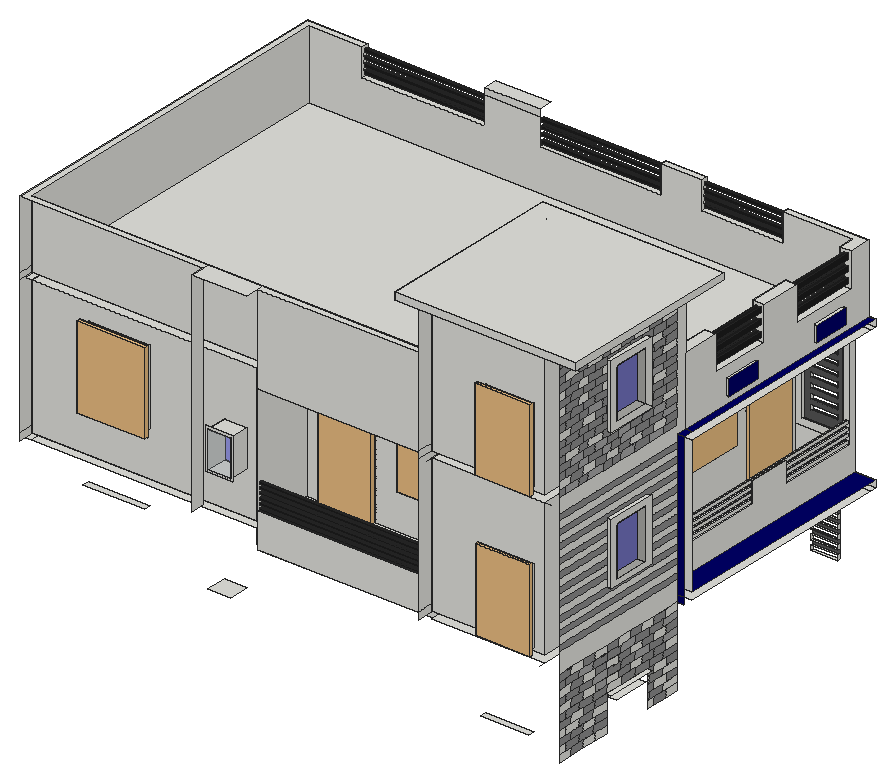
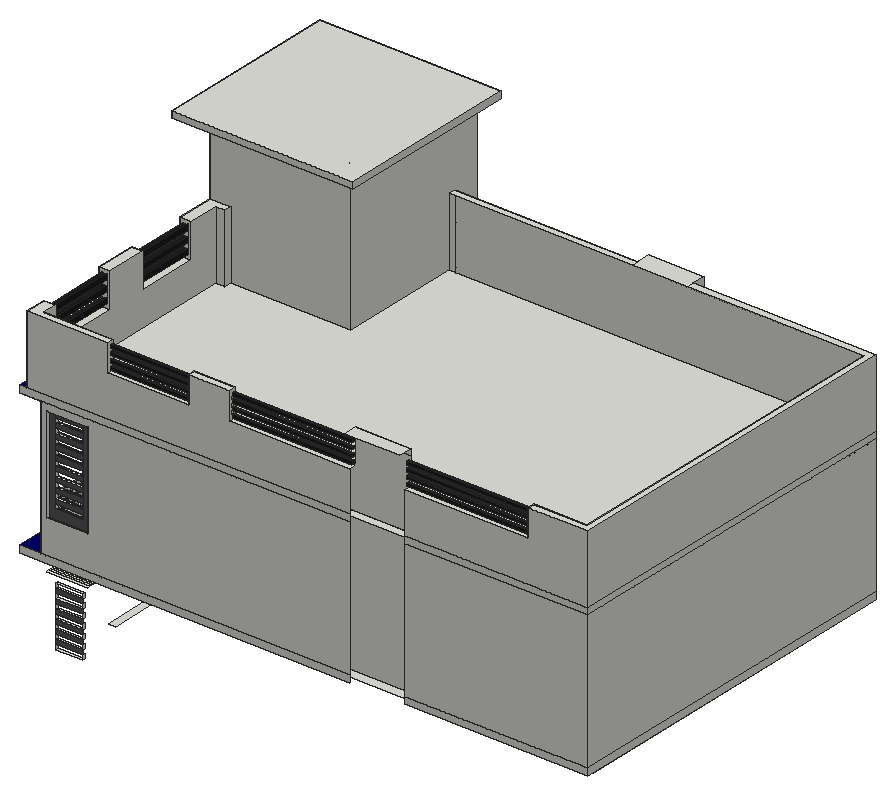
# SketchUp Ruby script. Lengths in inches.
U = 1.inch
M = Sketchup.active_model
def pt(a) = Geom::Point3d.new(a.map { |v| v * U })
def face(e, loops, mat)
  f = e.add_face(loops[0].map { |a| pt(a) })
  loops[1..].each { |l| e.add_face(l.map { |a| pt(a) }).erase! }
  f.material = f.back_material = mat if mat
  f
end
# faces: each face lists its corners as indices into pts; further lists are holes
def faces(e, pts, list, mat = nil) = list.each { |f| face(e, (f[0].is_a?(Array) ? f : [f]).map { |l| l.map { |i| pts[i] } }, mat) }
# xy, xz, yz: faces in a plane at the given z, y or x. An outline is a flat list of corners, or four numbers for a rectangle; further outlines are holes
def ring(l) = l.size == 4 ? [[l[0], l[1]], [l[2], l[1]], [l[2], l[3]], [l[0], l[3]]] : l.each_slice(2).to_a
def flat(e, list, mat, &to3) = list.each { |f| face(e, (f[0].is_a?(Array) ? f : [f]).map { |l| ring(l).map { |u, v| to3.(u, v) } }, mat) }
def xy(e, z, list, mat = nil) = flat(e, list, mat) { |x, y| [x, y, z] }
def xz(e, y, list, mat = nil) = flat(e, list, mat) { |x, z| [x, y, z] }
def yz(e, x, list, mat = nil) = flat(e, list, mat) { |y, z| [x, y, z] }
def lines(e, pts, list) = list.each { |a, b| e.add_line(pt(pts[a]), pt(pts[b])) }
# prism: a flat outline (further loops are holes) pulled along v
def prism(e, loops, v, mat = nil)
  f = face(e, loops, mat); d = Geom::Vector3d.new(v.map { |x| x * U })
  f.pushpull(f.normal.samedirection?(d) ? d.length : -d.length)
end
def box(e, o, s, mat = nil) = prism(e, [[o, [o[0] + s[0], o[1], o[2]], [o[0] + s[0], o[1] + s[1], o[2]], [o[0], o[1] + s[1], o[2]]]], [0, 0, s[2]], mat)
def at(x, y, z, deg = 0) = Geom::Transformation.translation(pt([x, y, z])) * Geom::Transformation.rotation(ORIGIN, Z_AXIS, deg.degrees)
def axes(o, x, y, z) = Geom::Transformation.new([*x, 0, *y, 0, *z, 0, *pt(o).to_a, 1])
def part(name) = M.definitions.add(name)
# library, detail: a bought-in or finely detailed component or shape, given as its bounding box
def library(name, o, s) = part(name).tap { |d| box(d.entities, o, s) }
def detail(e, o, s) = box(e.add_group.entities, o, s)
def put(e, d, t, mat = nil) = e.add_instance(d, t).tap { |i| i.material = mat if mat }
def group(e, t, mat = nil) = e.add_group.tap { |g| g.transformation = t; g.material = mat if mat }.entities
root = M.entities
M.materials.add("Glass_Basic_01").color = [0, 0, 0]
M.materials["Glass_Basic_01"].alpha = 0.25
M.materials.add("Glass_Basic_1").color = [161, 173, 186]
M.materials["Glass_Basic_1"].alpha = 0.25
M.materials.add("I02_Moonlit_Azure").color = [153, 153, 255]
M.materials.add("I08_Inkstorm").color = [0, 0, 102]
M.materials.add("M03_Pewter_Shine").color = [168, 168, 168]
M.materials.add("M04_Stone_Frost").color = [142, 142, 142]
M.materials.add("M06_Steel_Smoke").color = [86, 86, 86]
M.materials.add("M08_Obsidian_Black").color = [30, 30, 30]
c1 = library("porta+4",[0.2,-5.42,1.33],[46.55,4.72,83.21])
c2 = library("mesh-162",[-1607.75,-1245.64,-53.98],[1739.16,1702.88,120.91])
c3 = part("Group9")
put(c3.entities,c2,at(0,0,0))
c4 = part("Balcony railing")
xy(c4.entities,0.4,[[0,0.79,160.5,2.29]])
xy(c4.entities,2.4,[[0,0.79,160.5,2.29]])
xy(c4.entities,4.59,[[0,0.79,160.5,2.29]])
xy(c4.entities,6.59,[[0,0.79,160.5,2.29]])
xy(c4.entities,8.79,[[0,0.79,160.5,2.29]])
xy(c4.entities,10.79,[[0,0.79,160.5,2.29]])
xy(c4.entities,12.98,[[0,0.79,160.5,2.29]])
xy(c4.entities,14.98,[[0,0.79,160.5,2.29]])
xy(c4.entities,17.17,[[0,0.79,160.5,2.29]])
xy(c4.entities,19.17,[[0,0.79,160.5,2.29]])
xy(c4.entities,21.36,[[0,0.79,160.5,2.29]])
xy(c4.entities,23.36,[[0,0.79,160.5,2.29]])
xz(c4.entities,0.79,[[0,0.4,160.5,2.4],[0,4.59,160.5,6.59],[0,8.79,160.5,10.79],[0,12.98,160.5,14.98],[0,17.17,160.5,19.17],
  [0,21.36,160.5,23.36]])
xz(c4.entities,2.29,[[0,0.4,160.5,2.4],[0,4.59,160.5,6.59],[0,8.79,160.5,10.79],[0,12.98,160.5,14.98],[0,17.17,160.5,19.17],
  [0,21.36,160.5,23.36]])
yz(c4.entities,0,[[[0,0,3,24],[0.79,21.36,2.29,23.36],[0.79,17.17,2.29,19.17],[0.79,12.98,2.29,14.98],[0.79,8.79,2.29,10.79],[0.79,4.59,2.29,6.59],[0.79,0.4,2.29,2.4]]])
yz(c4.entities,160.5,[[0.79,0.4,2.29,2.4],[0.79,4.59,2.29,6.59],[0.79,8.79,2.29,10.79],[0.79,12.98,2.29,14.98],[0.79,17.17,2.29,19.17],
  [0.79,21.36,2.29,23.36]])
c5 = part("RAIL")
xy(c5.entities,0,[[0,0,2,195]])
xy(c5.entities,2.57,[[0,0,2,195]])
xy(c5.entities,5.14,[[0,0,2,195]])
xy(c5.entities,7.71,[[0,0,2,195]])
xy(c5.entities,10.29,[[0,0,2,195]])
xy(c5.entities,12.86,[[0,0,2,195]])
xy(c5.entities,15.43,[[0,0,2,195]])
xy(c5.entities,18,[[0,0,2,195]])
xz(c5.entities,0,[[0,2.57,2,5.14],[0,7.71,2,10.29],[0,12.86,2,15.43]])
xz(c5.entities,195,[[0,0,2,2.57],[0,5.14,2,7.71],[0,10.29,2,12.86],[0,15.43,2,18]])
yz(c5.entities,0,[[0,0,195,2.57],[0,5.14,195,7.71],[0,10.29,195,12.86],[0,15.43,195,18]])
yz(c5.entities,2,[[0,0,195,2.57],[0,5.14,195,7.71],[0,10.29,195,12.86],[0,15.43,195,18]])
c6 = library("mesh-160",[-91.39,-1008.79,-36.9],[2366.42,1739.16,65.81])
c7 = part("Group4")
g1 = group(c7.entities,at(-5.75,-6.15,0))
put(g1,c6,axes([0,0,0],[1,0,0],[0,0,1],[0,-1,0]))
c8 = library("mesh-166",[-1553.69,-2604.3125,-42.18],[1702.88,1401.6,88.28])
c9 = part("Group17")
put(c9.entities,c8,at(294.66,859.51,3.5))
xy(root,180,[[468,356,492,358]])
xy(root,184,[[468,356,492,358]])
xy(root,188,[[468,356,492,358]])
xy(root,189,[[447,21,489,27]])
xy(root,192,[[468,356,492,358]])
xy(root,196,[[198.5,33,218.5,51],[468,356,492,358]])
xy(root,200,[[468,356,492,358]])
xy(root,201.86,[[512,78.73,520,110.73]])
xy(root,204,[[468,356,492,358]])
xy(root,206,[[247.5,99,289.5,105]])
xy(root,207,[[319.5,95,361.5,105],[450,219,456,285],[450,303,456,345]])
xy(root,208,[[468,356,492,358]])
xy(root,208.2,[[516,72.6,520,117.43]])
xy(root,210,[[316.5,95,364.5,99]])
xy(root,212,[[468,356,492,358]])
xy(root,216,[[468,356,492,358]])
xy(root,220,[[468,356,492,358]])
xy(root,224,[[468,356,492,358]])
xy(root,228,[[468,356,492,358]])
xy(root,231,[[79.5,45,133.5,51]])
xy(root,232,[[468,356,492,358]])
xy(root,234,[[232.5,45,393,51]])
xy(root,240,[[462,354,498,356],[462,356,498,358],[462,358,498,360]])
xy(root,246,[[399,27,498,153],[24,51,30,354],[30,51,30,354,450,354,450,159,393,159,393,105,226.5,105,226.5,51],[232.5,51,393,99],[450,159,456,354],
  [456,159,522,354],[504,354,522,360]])
xy(root,252,[[399,27,498,27,498,153,450,153,450,354,30,354,30,51,226.5,51,226.5,105,399,105],[232.5,51,393,99],[456,159,498,354]])
xy(root,252,[[504,159,522,360]],"I08_Inkstorm")
xy(root,255,[[447,21,489,27],[247.5,99,289.5,105],[450,303,456,345]])
xy(root,264,[[232.5,45,393,51]])
xy(root,276,[[498,159,504,159,504,247.5,502.35,247.5,502.35,283.5,504,283.5,504,354,498,354]])
xy(root,282,[[462,354,498,356],[462,356,498,358],[462,358,498,360]])
xy(root,288,[[316.5,95,364.5,99]])
xy(root,290,[[198.5,33,218.5,51],[468,356,492,358]])
xy(root,291,[[79.5,45,133.5,51],[319.5,95,361.5,105],[450,219,456,285]])
xy(root,292.2,[[516,72.73,520,116.73]])
xy(root,294,[[502.35,247.5,504,283.5]])
xy(root,294.25,[[468,356,492,358]])
xy(root,296,[[512,78.73,520,110.73]])
xy(root,298.5,[[468,356,492,358]])
xy(root,302.75,[[468,356,492,358]])
xy(root,307,[[468,356,492,358]])
xy(root,311.25,[[468,356,492,358]])
xy(root,315.5,[[468,356,492,358]])
xy(root,319.75,[[468,356,492,358]])
xy(root,321,[[447,21,489,27]])
xy(root,322,[[198.5,33,218.5,51]])
xy(root,324,[[468,356,492,358]])
xy(root,328.25,[[468,356,492,358]])
xy(root,332.5,[[468,356,492,358]])
xy(root,333,[[319.5,95,361.5,105],[247.5,99,289.5,105],[450,219,456,285],[450,303,456,345]])
xy(root,336,[[316.5,95,364.5,99]])
xy(root,336.75,[[468,356,492,358]])
xy(root,340,[[512,78.73,520,110.73]])
xy(root,341,[[468,356,492,358]])
xy(root,345.25,[[468,356,492,358]])
xy(root,346.04,[[516,72.73,520,116.73]])
xy(root,349.5,[[468,356,492,358]])
xy(root,353.75,[[468,356,492,358]])
xy(root,357,[[79.5,45,133.5,51]])
xy(root,358,[[468,356,492,358]])
xy(root,360,[[232.5,45,393,51]])
xy(root,362,[[468,356,492,358]])
xy(root,366,[[462,354,498,356],[462,356,498,358],[462,358,498,360]])
xy(root,372,[[399,27,498,51],[24,51,30,360],[30,51,30,354,450,354,450,153,498,153,498,51,399,51,399,105,226.5,105,226.5,51],[232.5,51,393,99],[456,159,522,354],
  [504,354,522,360]])
xy(root,378,[[399,27,498,153],[30,51,393,51,393,159,498,159,498,165,506.09,165,506.09,354,30,354]])
xy(root,378,[[516,150,522,159],[516,159,522,360]],"I08_Inkstorm")
xy(root,381,[[447,21,489,27]])
xy(root,385.3125,[[516,203.09,519,235.03],[516,299.09,519,331.03]])
xy(root,398.86,[[516,203.09,519,235.03],[516,299.09,519,331.03]])
xy(root,408,[[506.09,192.5,516,245],[506.09,281,516,341]])
xy(root,411,[[509.09,192.5,513,245],[509.09,281,513,341]])
xy(root,414,[[76.5,354,184.5,360],[232.5,354,338.25,360],[374.25,354,445.125,360]])
xy(root,414.5,[[516,72.73,520,116.73]])
xy(root,415.8,[[509.09,192.5,513,245],[509.09,281,513,341]],"M08_Obsidian_Black")
xy(root,416,[[76.5,356,184.5,358],[232.5,356,338.25,358],[374.25,356,445.125,358]])
xy(root,418.86,[[76.5,356,184.5,358],[232.5,356,338.25,358],[374.25,356,445.125,358]],"M08_Obsidian_Black")
xy(root,420.5,[[512,78.73,520,110.73]])
xy(root,420.6,[[509.09,192.5,513,245],[509.09,281,513,341]])
xy(root,421.71,[[76.5,356,184.5,358],[232.5,356,338.25,358],[374.25,356,445.125,358]])
xy(root,424.57,[[76.5,356,184.5,358],[232.5,356,338.25,358],[374.25,356,445.125,358]],"M08_Obsidian_Black")
xy(root,425.4,[[509.09,192.5,513,245],[509.09,281,513,341]],"M08_Obsidian_Black")
xy(root,427.43,[[76.5,356,184.5,358],[232.5,356,338.25,358],[374.25,356,445.125,358]])
xy(root,430.2,[[509.09,192.5,513,245],[509.09,281,513,341]])
xy(root,430.29,[[76.5,356,184.5,358],[232.5,356,338.25,358],[374.25,356,445.125,358]],"M08_Obsidian_Black")
xy(root,433.14,[[76.5,356,184.5,358],[232.5,356,338.25,358],[374.25,356,445.125,358]])
xy(root,435,[[509.09,192.5,513,245],[509.09,281,513,341]],"M08_Obsidian_Black")
xy(root,436,[[76.5,356,184.5,358],[232.5,356,338.25,358],[374.25,356,445.125,358]],"M08_Obsidian_Black")
xy(root,438,[[184.5,33,232.5,51],[24,45,184.5,45,184.5,51,30,51,30,354,76.5,354,76.5,360,24,360],[232.5,45,393,51],[498,159,516,159,516,192.5,506.09,192.5,506.09,165,498,165],[506.09,245,516,281],
  [506.09,341,516,341,516,360,445.125,360,445.125,354,506.09,354],[338.25,354,374.25,360]])
xy(root,444,[[184.5,354,232.5,366]])
xy(root,447,[[447,21,489,27]])
xy(root,464.5,[[512,78.73,520,110.73]])
xy(root,470.5,[[516,72.73,520,116.73]])
xy(root,498,[[[381,9,540,171],[393,21,516,159]],[393,21,516,27],[393,27,399,159],[399,27,498,153],[498,27,516,159],
  [399,153,498,159]])
xy(root,504,[[381,9,540,171]])
xz(root,9,[[381,498,540,504]])
xz(root,21,[[[444,252,492,324],[447,255,489,321]],[[444,378,492,450],[447,381,489,447]]])
xz(root,27,[[[399,252,498,372],[447,255,489,321]],[[399,378,498,498],[447,381,489,447]]])
xz(root,33,[[[196.5,288,220.5,324],[198.5,290,218.5,322]]])
xz(root,33,[[198.5,290,218.5,322]],"Glass_Basic_1")
xz(root,45,[[232.5,234,393,264],[[76.5,288,136.5,360],[79.5,291,133.5,357]],[232.5,360,393,438]])
xz(root,51,[[232.5,234,393,246],[[30,252,226.5,372],[79.5,291,133.5,357],[198.5,290,218.5,322]],[232.5,252,393,264],[232.5,360,393,372],[30,378,387,438],
  [387,378,393,438]])
xz(root,51,[[198.5,290,218.5,322]],"I02_Moonlit_Azure")
xz(root,72.73,[[516,292.2,520,346.04],[516,414.5,520,470.5]])
xz(root,78.73,[[512,296,520,340],[512,420.5,520,464.5]])
xz(root,95,[[[316.5,288,364.5,336],[319.5,291,361.5,333]]])
xz(root,99,[[[232.5,252,244.5,252,244.5,336,292.5,336,292.5,252,393,252,393,372,232.5,372],[316.5,288,364.5,336]],[[244.5,252,292.5,336],[247.5,255,289.5,333]]])
xz(root,105,[[[226.5,252,393,372],[247.5,255,289.5,333],[319.5,291,361.5,333]],[393,252,399,372]])
xz(root,110.73,[[512,296,520,340],[512,420.5,520,464.5]])
xz(root,116.73,[[516,292.2,520,346.04],[516,414.5,520,470.5]])
xz(root,150,[[516,246,522,252],[516,252,522,378]],"I08_Inkstorm")
xz(root,153,[[450,252,498,372],[399,378,498,498]])
xz(root,159,[[456,252,456,372,522,372,522,252,504,252,504,276,498,276,498,252],[393,378,393,498,516,498,516,438,498,438,498,378]])
xz(root,165,[[498,378,506.09,438]])
xz(root,171,[[381,498,540,504]])
xz(root,192.5,[[[506.09,408,516,438],[509.09,411,513,435]],[509.09,415.8,513,420.6],[509.09,425.4,513,430.2]])
xz(root,203.09,[[516,385.3125,519,398.86]])
xz(root,219,[[450,291,456,333]])
xz(root,235.03,[[516,385.3125,519,398.86]])
xz(root,245,[[[506.09,408,516,438],[509.09,430.2,513,435],[509.09,411,513,415.8],[509.09,420.6,513,425.4]]])
xz(root,247.5,[[502.35,276,504,294]])
xz(root,281,[[[506.09,408,516,438],[509.09,411,513,435]],[509.09,415.8,513,420.6],[509.09,425.4,513,430.2]])
xz(root,283.5,[[502.35,276,504,294]])
xz(root,285,[[450,291,456,333]])
xz(root,299.09,[[516,385.3125,519,398.86]])
xz(root,303,[[450,255,456,333]])
xz(root,331.03,[[516,385.3125,519,398.86]])
xz(root,341,[[[506.09,408,516,438],[509.09,430.2,513,435],[509.09,411,513,415.8],[509.09,420.6,513,425.4]]])
xz(root,345,[[450,255,456,333]])
xz(root,354,[[30,252,450,372],[456,252,498,276],[[456,276,504,372],[462,282,498,366]],[30,378,506.09,378,506.09,438,445.125,438,445.125,414,374.25,414,374.25,438,338.25,438,338.25,414,232.5,414,232.5,438,184.5,438,184.5,414,76.5,414,76.5,438,30,438],[184.5,438,232.5,444]])
xz(root,356,[[[462,282,498,366],[468,290,492,294.25],[468,298.5,492,302.75],[468,307,492,311.25],[468,315.5,492,319.75],[468,324,492,328.25],[468,332.5,492,336.75],[468,341,492,345.25],[468,349.5,492,353.75],[468,358,492,362]]],"M06_Steel_Smoke")
xz(root,356,[[76.5,416,184.5,418.86],[232.5,416,338.25,418.86],[374.25,416,445.125,418.86],[76.5,421.71,184.5,424.57],[232.5,421.71,338.25,424.57],
  [374.25,421.71,445.125,424.57],[76.5,427.43,184.5,430.29],[232.5,427.43,338.25,430.29],[374.25,427.43,445.125,430.29],[76.5,433.14,184.5,436],
  [232.5,433.14,338.25,436],[374.25,433.14,445.125,436]],"M08_Obsidian_Black")
xz(root,358,[[468,184,492,188],[468,192,492,196],[468,200,492,204],[468,208,492,212],[468,216,492,220],
  [468,224,492,228],[[462,282,498,366],[468,290,492,362]],[468,294.25,492,298.5],[468,302.75,492,307],[468,311.25,492,315.5],
  [468,319.75,492,324],[468,328.25,492,332.5],[468,336.75,492,341],[468,345.25,492,349.5],[468,353.75,492,358]],"M06_Steel_Smoke")
xz(root,358,[[76.5,416,184.5,418.86],[232.5,416,338.25,418.86],[374.25,416,445.125,418.86],[76.5,421.71,184.5,424.57],[232.5,421.71,338.25,424.57],
  [374.25,421.71,445.125,424.57],[76.5,427.43,184.5,430.29],[232.5,427.43,338.25,430.29],[374.25,427.43,445.125,430.29],[76.5,433.14,184.5,436],
  [232.5,433.14,338.25,436],[374.25,433.14,445.125,436]],"M08_Obsidian_Black")
xz(root,360,[[24,246,184.5,252],[232.5,246,522,252],[24,252,184.5,372],[[232.5,252,504,372],[462,282,498,366]],[24,372,184.5,378],
  [232.5,372,522,378],[24,378,24,438,76.5,438,76.5,414,184.5,414,184.5,378],[232.5,378,232.5,414,338.25,414,338.25,438,374.25,438,374.25,414,445.125,414,445.125,438,516,438,516,378]])
yz(root,24,[[45,246,360,252],[45,252,360,372],[45,372,360,378],[45,378,360,438]])
yz(root,30,[[51,252,354,372],[51,378,354,438]])
yz(root,76.5,[[[354,414,360,438],[356,416,358,436]],[356,418.86,358,421.71],[356,424.57,358,427.43],[356,430.29,358,433.14]])
yz(root,79.5,[[45,291,51,357]])
yz(root,133.5,[[45,291,51,357]])
yz(root,184.5,[[33,252,45,438]])
yz(root,198.5,[[33,290,51,322]])
yz(root,218.5,[[33,290,51,322]])
yz(root,226.5,[[51,234,105,246],[51,252,105,264],[51,264,105,360],[51,360,105,372]])
yz(root,232.5,[[51,252,99,252,99,372,51,372,51,360,45,360,45,264,51,264]])
yz(root,247.5,[[99,255,105,333]])
yz(root,289.5,[[99,255,105,333]])
yz(root,316.5,[[95,288,99,336]])
yz(root,319.5,[[95,291,105,333]])
yz(root,338.25,[[[354,414,360,438],[356,416,358,436]],[356,418.86,358,421.71],[356,424.57,358,427.43],[356,430.29,358,433.14]])
yz(root,361.5,[[95,291,105,333]])
yz(root,364.5,[[95,288,99,336]])
yz(root,374.25,[[[354,414,360,438],[356,416,358,436]],[356,418.86,358,421.71],[356,424.57,358,427.43],[356,430.29,358,433.14]])
yz(root,381,[[9,498,171,504]])
yz(root,393,[[45,234,51,246],[21,246,45,252],[21,252,45,372],[51,252,51,264,45,264,45,360,51,360,51,372,99,372,99,252],[21,372,45,378],
  [21,378,21,498,159,498,159,378,51,378,51,438,45,438,45,378]])
yz(root,399,[[27,252,105,372],[27,378,153,498]])
yz(root,445.125,[[[354,414,360,438],[356,433.14,358,436],[356,427.43,358,430.29],[356,421.71,358,424.57],[356,416,358,418.86]]])
yz(root,447,[[21,255,27,321],[21,381,27,447]])
yz(root,450,[[[153,252,354,372],[303,255,345,333],[219,291,285,333]]])
yz(root,456,[[[159,252,300,252,300,336,348,336,348,252,354,252,354,372,159,372],[216,288,288,336]],[[300,252,348,336],[303,255,345,333]],[[216,288,288,336],[219,291,285,333]]])
yz(root,462,[[354,282,356,366],[358,282,360,366]])
yz(root,468,[[356,180,358,184],[356,188,358,192],[356,196,358,200],[356,204,358,208],[356,212,358,216],
  [356,220,358,224],[356,228,358,232],[356,290,358,294.25],[356,298.5,358,302.75],[356,307,358,311.25],
  [356,315.5,358,319.75],[356,324,358,328.25],[356,332.5,358,336.75],[356,341,358,345.25],[356,349.5,358,353.75],
  [356,358,358,362]])
yz(root,489,[[21,255,27,321],[21,381,27,447]])
yz(root,492,[[356,180,358,184],[356,188,358,192],[356,196,358,200],[356,204,358,208],[356,212,358,216],
  [356,220,358,224],[356,228,358,232],[356,290,358,294.25],[356,298.5,358,302.75],[356,307,358,311.25],
  [356,315.5,358,319.75],[356,324,358,328.25],[356,332.5,358,336.75],[356,341,358,345.25],[356,349.5,358,353.75],
  [356,358,358,362]])
yz(root,498,[[27,252,153,372],[159,252,354,276],[354,282,356,366],[358,282,360,366],[27,378,153,498],
  [159,378,165,438]])
yz(root,502.35,[[247.5,276,283.5,294]])
yz(root,504,[[159,252,360,252,360,372,354,372,354,276,283.5,276,283.5,294,247.5,294,247.5,276,159,276]])
yz(root,506.09,[[165,378,165,438,192.5,438,192.5,408,245,408,245,438,281,438,281,408,341,408,341,438,354,438,354,378]])
yz(root,509.09,[[192.5,411,245,415.8],[281,411,341,415.8],[192.5,420.6,245,425.4],[281,420.6,341,425.4],[192.5,430.2,245,435],
  [281,430.2,341,435]],"M08_Obsidian_Black")
yz(root,512,[[78.73,296,110.73,340],[78.73,420.5,110.73,464.5]],"I02_Moonlit_Azure")
yz(root,513,[[192.5,411,245,415.8],[281,411,341,415.8],[192.5,420.6,245,425.4],[281,420.6,341,425.4],[192.5,430.2,245,435],
  [281,430.2,341,435]],"M08_Obsidian_Black")
yz(root,516,[[21,176.7,33.9,183],[46.8,176.7,59.7,183],[59.7,176.7,72.6,183],[117.43,176.7,124.2,183],[137.1,176.7,150,183],
  [21,183,27.45,189.3],[72.6,183,73.41,189.3],[134.68,183,150,189.3],[46.8,189.3,59.7,195.6],[124.2,189.3,137.1,195.6],
  [21,195.6,27.45,201.9],[27.45,195.6,42.77,201.9],[58.09,195.6,72.6,201.9],[117.43,195.6,119.36,201.9],[134.68,195.6,150,201.9],
  [33.9,201.9,46.8,208.2],[124.2,201.9,137.1,208.2],[73.41,208.2,88.72,214.5],[21,214.5,33.9,220.8],[46.8,214.5,59.7,220.8],
  [72.6,214.5,85.5,220.8],[98.4,214.5,111.3,220.8],[137.1,214.5,150,220.8],[21,227.1,33.9,233.4],[46.8,227.1,59.7,233.4],
  [72.6,227.1,85.5,233.4],[98.4,227.1,111.3,233.4],[124.2,227.1,137.1,233.4],[33.9,239.7,46.8,246],[59.7,239.7,72.6,246],
  [85.5,239.7,98.4,246],[111.3,239.7,124.2,246],[137.1,239.7,150,246],[21,246,150,263.7],[21,269.4,150,275.1],
  [21,280.8,150,286.5],[21,292.2,72.73,297.9],[116.73,292.2,150,297.9],[21,303.6,72.73,309.3],[116.73,303.6,150,309.3],
  [21,315,72.73,320.7],[116.73,315,150,320.7],[21,326.4,72.73,332.1],[116.73,326.4,150,332.1],[21,337.8,72.73,343.5],
  [116.73,337.8,150,343.5],[21,349.2,150,354.9],[21,360.6,150,366.3],[21,372,150,372,150,378,159,378,159,498,150,498,150,384.6,21,384.6],[[159,378,360,378,360,438,341,438,341,408,281,408,281,438,245,438,245,408,192.5,408,192.5,438,159,438],[203.09,385.3125,235.03,398.86],[299.09,385.3125,331.03,398.86]],
  [21,390.9,33.9,397.2],[46.8,390.9,59.7,397.2],[72.6,390.9,85.5,397.2],[98.4,390.9,111.3,397.2],[124.2,390.9,137.1,397.2],
  [27.45,409.8,42.77,416.1],[52.44,409.8,68.36,416.1],[76.73,409.8,88.72,414.5],[104.04,409.8,119.36,409.8,119.36,416.1,116.73,416.1,116.73,414.5,104.04,414.5],[134.68,409.8,150,416.1],
  [21,428.7,33.9,435],[46.8,428.7,59.7,435],[72.6,428.7,72.73,435],[124.2,428.7,137.1,435],[21,447.6,27.45,453.9],
  [42.77,447.6,52.44,453.9],[68.36,447.6,72.73,453.9],[116.73,447.6,119.36,453.9],[134.68,447.6,150,453.9],[21,460.2,27.45,466.5],
  [42.77,460.2,52.44,466.5],[68.36,460.2,72.73,466.5],[119.36,460.2,134.68,466.5],[27.45,472.8,42.77,479.1],[52.44,472.8,68.36,479.1],
  [76.73,472.8,88.72,479.1],[104.04,472.8,119.36,479.1],[134.68,472.8,150,479.1],[33.9,491.7,46.8,498],[59.7,491.7,72.6,498],
  [85.5,491.7,98.4,498],[111.3,491.7,124.2,498],[137.1,491.7,150,498]])
yz(root,516,[[59.7,214.5,72.6,220.8],[58.09,220.8,73.41,227.1],[104.04,220.8,119.36,227.1],[134.68,220.8,150,227.1],[42.77,233.4,58.09,239.7],
  [88.72,233.4,104.04,239.7],[134.68,233.4,150,239.7],[27.45,384.6,42.77,390.9],[52.44,384.6,69.72,390.9],[88.72,384.6,104.04,390.9],
  [119.36,384.6,134.68,390.9],[42.77,397.2,52.44,403.5],[68.36,397.2,76.73,403.5],[88.72,397.2,104.04,403.5],[134.68,397.2,150,403.5],
  [33.9,403.5,46.8,409.8],[59.7,403.5,72.6,409.8],[85.5,403.5,98.4,409.8],[124.2,403.5,137.1,409.8],[52.44,435,68.36,441.3],
  [119.36,435,134.68,441.3],[33.9,479.1,46.8,485.4],[85.5,479.1,98.4,485.4],[98.4,479.1,111.3,485.4],[52.44,485.4,68.36,491.7],
  [119.36,485.4,134.68,491.7]],"M03_Pewter_Shine")
yz(root,516,[[33.9,176.7,46.8,183],[124.2,176.7,137.1,183],[27.45,183,42.77,189.3],[42.77,183,58.09,189.3],[58.09,183,72.6,189.3],
  [117.43,183,119.36,189.3],[119.36,183,134.68,189.3],[21,189.3,33.9,195.6],[33.9,189.3,46.8,195.6],[59.7,189.3,72.6,195.6],
  [117.43,189.3,124.2,195.6],[137.1,189.3,150,195.6],[42.77,195.6,58.09,201.9],[72.6,195.6,73.41,201.9],[119.36,195.6,134.68,201.9],
  [21,201.9,33.9,208.2],[46.8,201.9,59.7,208.2],[59.7,201.9,72.6,208.2],[117.43,201.9,124.2,208.2],[137.1,201.9,150,208.2],
  [21,208.2,27.45,214.5],[27.45,208.2,42.77,214.5],[42.77,208.2,58.09,214.5],[58.09,208.2,73.41,214.5],[88.72,208.2,104.04,214.5],
  [104.04,208.2,119.36,214.5],[119.36,208.2,134.68,214.5],[134.68,208.2,150,214.5],[33.9,214.5,46.8,220.8],[85.5,214.5,98.4,220.8],
  [111.3,214.5,124.2,220.8],[124.2,214.5,137.1,220.8],[21,220.8,27.45,227.1],[27.45,220.8,42.77,227.1],[42.77,220.8,58.09,227.1],
  [73.41,220.8,88.72,227.1],[88.72,220.8,104.04,227.1],[119.36,220.8,134.68,227.1],[33.9,227.1,46.8,233.4],[59.7,227.1,72.6,233.4],
  [85.5,227.1,98.4,233.4],[111.3,227.1,124.2,233.4],[137.1,227.1,150,233.4],[21,233.4,27.45,239.7],[27.45,233.4,42.77,239.7],
  [58.09,233.4,73.41,239.7],[73.41,233.4,88.72,239.7],[104.04,233.4,119.36,239.7],[119.36,233.4,134.68,239.7],[21,239.7,33.9,246],
  [46.8,239.7,59.7,246],[72.6,239.7,85.5,246],[98.4,239.7,111.3,246],[124.2,239.7,137.1,246],[21,263.7,150,269.4],
  [21,275.1,150,280.8],[21,286.5,150,292.2],[21,297.9,72.73,303.6],[116.73,297.9,150,303.6],[21,309.3,72.73,315],
  [116.73,309.3,150,315],[21,320.7,72.73,326.4],[116.73,320.7,150,326.4],[21,332.1,72.73,337.8],[116.73,332.1,150,337.8],
  [21,343.5,72.73,343.5,72.73,346.04,116.73,346.04,116.73,343.5,150,343.5,150,349.2,21,349.2],[21,354.9,150,360.6],[21,366.3,150,372],[21,384.6,27.45,390.9],[42.77,384.6,52.44,390.9],
  [69.72,384.6,78.09,390.9],[78.09,384.6,88.72,390.9],[104.04,384.6,119.36,390.9],[134.68,384.6,150,390.9],[33.9,390.9,46.8,397.2],
  [59.7,390.9,72.6,397.2],[85.5,390.9,98.4,397.2],[111.3,390.9,124.2,397.2],[137.1,390.9,150,397.2],[21,397.2,27.45,403.5],
  [27.45,397.2,42.77,403.5],[52.44,397.2,68.36,403.5],[76.73,397.2,88.72,403.5],[104.04,397.2,119.36,403.5],[119.36,397.2,134.68,403.5],
  [21,403.5,33.9,409.8],[46.8,403.5,59.7,409.8],[72.6,403.5,85.5,409.8],[98.4,403.5,111.3,409.8],[111.3,403.5,124.2,409.8],
  [137.1,403.5,150,409.8],[21,409.8,27.45,416.1],[42.77,409.8,52.44,416.1],[68.36,409.8,76.73,409.8,76.73,414.5,72.73,414.5,72.73,416.1,68.36,416.1],[88.72,409.8,104.04,414.5],
  [119.36,409.8,134.68,416.1],[21,416.1,33.9,422.4],[33.9,416.1,46.8,422.4],[46.8,416.1,59.7,422.4],[59.7,416.1,72.6,422.4],
  [72.6,416.1,72.73,422.4],[116.73,416.1,124.2,422.4],[124.2,416.1,137.1,422.4],[137.1,416.1,150,422.4],[21,422.4,27.45,428.7],
  [27.45,422.4,42.77,428.7],[42.77,422.4,52.44,428.7],[52.44,422.4,68.36,428.7],[68.36,422.4,72.73,428.7],[116.73,422.4,119.36,428.7],
  [119.36,422.4,134.68,428.7],[134.68,422.4,150,428.7],[33.9,428.7,46.8,435],[59.7,428.7,72.6,435],[116.73,428.7,124.2,435],
  [137.1,428.7,150,435],[21,435,27.45,441.3],[27.45,435,42.77,441.3],[42.77,435,52.44,441.3],[68.36,435,72.73,441.3],
  [116.73,435,119.36,441.3],[134.68,435,150,441.3],[21,441.3,33.9,447.6],[33.9,441.3,46.8,447.6],[46.8,441.3,59.7,447.6],
  [59.7,441.3,72.6,447.6],[72.6,441.3,72.73,447.6],[116.73,441.3,124.2,447.6],[124.2,441.3,137.1,447.6],[137.1,441.3,150,447.6],
  [27.45,447.6,42.77,453.9],[52.44,447.6,68.36,453.9],[119.36,447.6,134.68,453.9],[21,453.9,33.9,460.2],[33.9,453.9,46.8,460.2],
  [46.8,453.9,59.7,460.2],[59.7,453.9,72.6,460.2],[72.6,453.9,72.73,460.2],[116.73,453.9,124.2,460.2],[124.2,453.9,137.1,460.2],
  [137.1,453.9,150,460.2],[27.45,460.2,42.77,466.5],[52.44,460.2,68.36,466.5],[116.73,460.2,119.36,466.5],[134.68,460.2,150,466.5],
  [21,466.5,33.9,472.8],[33.9,466.5,46.8,472.8],[46.8,466.5,59.7,472.8],[59.7,466.5,72.6,472.8],[72.6,466.5,72.73,466.5,72.73,470.5,85.5,470.5,85.5,472.8,72.6,472.8],
  [116.73,466.5,124.2,466.5,124.2,472.8,111.3,472.8,111.3,470.5,116.73,470.5],[124.2,466.5,137.1,472.8],[137.1,466.5,150,472.8],[85.5,470.5,98.4,472.8],[98.4,470.5,111.3,472.8],
  [21,472.8,27.45,479.1],[42.77,472.8,52.44,479.1],[68.36,472.8,76.73,479.1],[88.72,472.8,104.04,479.1],[119.36,472.8,134.68,479.1],
  [21,479.1,33.9,485.4],[46.8,479.1,59.7,485.4],[59.7,479.1,72.6,485.4],[72.6,479.1,85.5,485.4],[111.3,479.1,124.2,485.4],
  [124.2,479.1,137.1,485.4],[137.1,479.1,150,485.4],[21,485.4,27.45,491.7],[27.45,485.4,42.77,491.7],[42.77,485.4,52.44,491.7],
  [68.36,485.4,76.73,491.7],[76.73,485.4,88.72,491.7],[88.72,485.4,104.04,491.7],[104.04,485.4,119.36,491.7],[134.68,485.4,150,491.7],
  [21,491.7,33.9,498],[46.8,491.7,59.7,498],[72.6,491.7,85.5,498],[98.4,491.7,111.3,498],[124.2,491.7,137.1,498]],"M04_Stone_Frost")
yz(root,519,[[203.09,385.3125,235.03,398.86],[299.09,385.3125,331.03,398.86]],"I08_Inkstorm")
yz(root,520,[[[72.73,292.2,116.73,346.04],[78.73,296,110.73,340]],[[72.73,414.5,116.73,470.5],[78.73,420.5,110.73,464.5]]])
yz(root,520,[[78.73,296,110.73,340],[78.73,420.5,110.73,464.5]],"Glass_Basic_01")
yz(root,540,[[9,498,171,504]])
p = [[498,153,246],[504,153,246],[498,27,246],[498,21,246],[450,354,372],[456,354,372],
  [399,27,372],[399,21,372],[498,27,372],[504,27,372],[498,153,372],[504,153,372],
  [498,51,372],[504,51,372],[399,153,504],[399,153,504.95],[520,110.73,420.5],[526,110.73,420.5],
  [456,354,246],[456,360,246],[456,360,372]]
lines(root,p,[[0,1],[2,3],[4,5],[6,7],[8,9],[10,11],[12,13],[14,15],[16,17],[18,19],[5,20]])
put(root,c1,at(244.3,100.84,250.63))
put(root,c1,at(454.16,299.8,250.63,90))
put(root,c3,axes([456.74,20.63,318.8],[0,0,0.04145],[-0.02786,0,0],[0,-0.02087,0]))
put(root,c4,at(232.5,45,264),"M08_Obsidian_Black")
put(root,c5,at(500.35,159,276))
put(root,c7,axes([456.7,218.96,315.87],[0,0.03043,0],[-0.02283,0,0],[0,0,0.02763]))
put(root,c9,axes([328.91,93.61,347.7],[-0.02795,0,0],[0,0,0.0341],[0,0.02795,0]))
put(root,c9,axes([92.05,43.05,377.57],[-0.03504,0,0],[0,0,0.05118],[0,0.03937,0]))
put(root,c3,axes([456.875,20.4375,444.81],[0,0,0.04142],[-0.02816,0,0],[0,-0.02441,0]))
